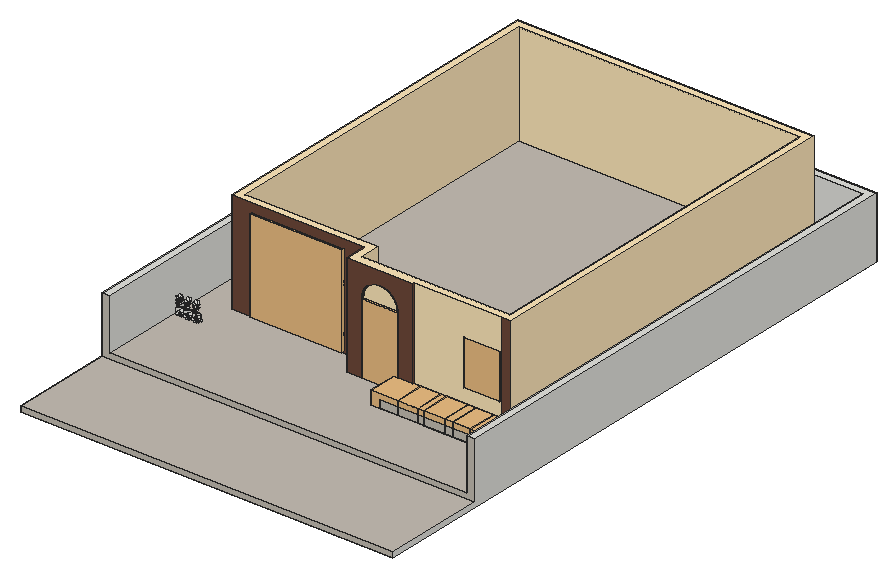
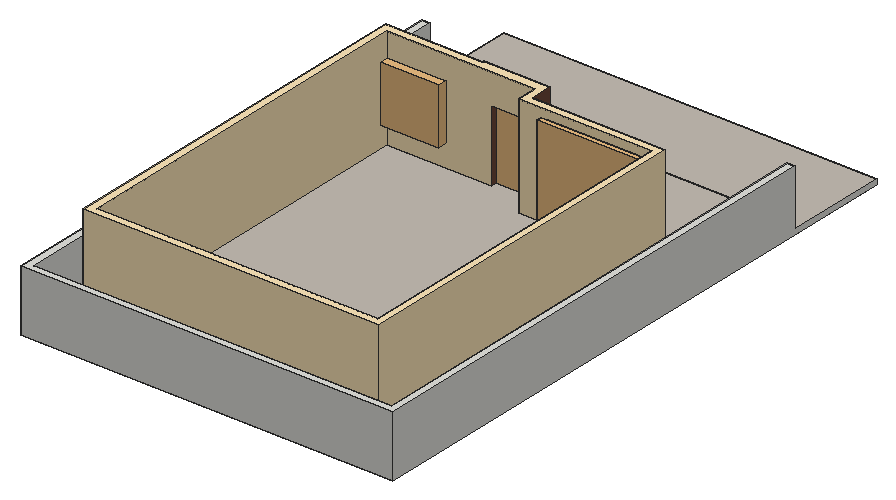
# SketchUp Ruby script. Lengths in inches.
U = 1.inch
M = Sketchup.active_model
def pt(a) = Geom::Point3d.new(a.map { |v| v * U })
def face(e, loops, mat)
  f = e.add_face(loops[0].map { |a| pt(a) })
  loops[1..].each { |l| e.add_face(l.map { |a| pt(a) }).erase! }
  f.material = f.back_material = mat if mat
  f
end
# faces: each face lists its corners as indices into pts; further lists are holes
def faces(e, pts, list, mat = nil) = list.each { |f| face(e, (f[0].is_a?(Array) ? f : [f]).map { |l| l.map { |i| pts[i] } }, mat) }
# xy, xz, yz: faces in a plane at the given z, y or x. An outline is a flat list of corners, or four numbers for a rectangle; further outlines are holes
def ring(l) = l.size == 4 ? [[l[0], l[1]], [l[2], l[1]], [l[2], l[3]], [l[0], l[3]]] : l.each_slice(2).to_a
def flat(e, list, mat, &to3) = list.each { |f| face(e, (f[0].is_a?(Array) ? f : [f]).map { |l| ring(l).map { |u, v| to3.(u, v) } }, mat) }
def xy(e, z, list, mat = nil) = flat(e, list, mat) { |x, y| [x, y, z] }
def xz(e, y, list, mat = nil) = flat(e, list, mat) { |x, z| [x, y, z] }
def yz(e, x, list, mat = nil) = flat(e, list, mat) { |y, z| [x, y, z] }
def lines(e, pts, list) = list.each { |a, b| e.add_line(pt(pts[a]), pt(pts[b])) }
# prism: a flat outline (further loops are holes) pulled along v
def prism(e, loops, v, mat = nil)
  f = face(e, loops, mat); d = Geom::Vector3d.new(v.map { |x| x * U })
  f.pushpull(f.normal.samedirection?(d) ? d.length : -d.length)
end
def box(e, o, s, mat = nil) = prism(e, [[o, [o[0] + s[0], o[1], o[2]], [o[0] + s[0], o[1] + s[1], o[2]], [o[0], o[1] + s[1], o[2]]]], [0, 0, s[2]], mat)
def at(x, y, z, deg = 0) = Geom::Transformation.translation(pt([x, y, z])) * Geom::Transformation.rotation(ORIGIN, Z_AXIS, deg.degrees)
def axes(o, x, y, z) = Geom::Transformation.new([*x, 0, *y, 0, *z, 0, *pt(o).to_a, 1])
def part(name) = M.definitions.add(name)
# library, detail: a bought-in or finely detailed component or shape, given as its bounding box
def library(name, o, s) = part(name).tap { |d| box(d.entities, o, s) }
def detail(e, o, s) = box(e.add_group.entities, o, s)
def put(e, d, t, mat = nil) = e.add_instance(d, t).tap { |i| i.material = mat if mat }
def group(e, t, mat = nil) = e.add_group.tap { |g| g.transformation = t; g.material = mat if mat }.entities
root = M.entities
M.materials.add("1026 AP 7946 SUNNY SIDE UP").color = [254, 231, 186]
M.materials.add("1916 AP K226 Macadamia Cream-N").color = [109, 72, 58]
M.materials.add("[Field Rectangle Tile]").color = [196, 189, 179]
M.materials.add("[Steel Brushed Stainless]").color = [48, 48, 48]
c1 = part("Component\#6")
p = [[0.01,0,0],[0,3.24,4.54],[4.32,3.24,4.54],[4.33,0,0]]
faces(c1.entities,p,[[0,1,2,3]])
c2 = library("porta 4",[0.2,-5.42,1.33],[46.55,4.72,83.21])
c3 = library("Glazed double door",[0,0,0],[5.31,78.43,99.16])
c4 = library("Curtains",[0,0,0],[101.19,6.19,107.53])
c5 = library("---------1\#1",[5.49,6.625,-77.21],[69.81,13.39,114.05])
c6 = library("Monstera",[-45.82,-31.79,6.14],[177.56,112.18,50.31])
c7 = library("Group\#26",[0,-3.33,0],[108,3.74,108])
xy(root,-12,[[0,0,438,710]])
xy(root,-6,[[0,0,438,120]],"[Field Rectangle Tile]")
xy(root,0,[[9,120,429,701]],"[Field Rectangle Tile]")
xy(root,60,[[0,120,9,120,9,701,429,701,429,120,438,120,438,710,0,710]])
xz(root,0,[[0,-12,438,-6]],"[Field Rectangle Tile]")
xz(root,120,[[0,-6,438,-6,438,60,429,60,429,0,9,0,9,60,0,60]],"[Field Rectangle Tile]")
xz(root,701,[[9,0,429,60]])
xz(root,710,[[0,-12,438,60]])
yz(root,0,[[0,-12,0,-6,120,-6,120,60,710,60,710,-12]])
yz(root,9,[[120,0,701,60]])
yz(root,429,[[120,0,701,60]])
yz(root,438,[[0,-12,710,-12,710,60,120,60,120,-6,0,-6]])
put(root,c1,axes([14.53,209.94,4.23],[-0.07499,0.16237,1.17608],[0.09639,1.17545,-0.15681],[1.25477,-0.08059,0.08234]))
put(root,c1,axes([28.31,209.94,4.23],[0.07499,0.16237,1.17608],[-0.09639,1.17545,-0.15681],[-1.25477,-0.08059,0.08234]))
put(root,c1,axes([24.34,209.94,4.23],[-0.07499,0.16237,1.17608],[0.09639,1.17545,-0.15681],[1.25477,-0.08059,0.08234]))
put(root,c1,axes([38.11,209.94,4.23],[0.07499,0.16237,1.17608],[-0.09639,1.17545,-0.15681],[-1.25477,-0.08059,0.08234]))
put(root,c1,axes([34.14,209.94,4.23],[-0.07499,0.16237,1.17608],[0.09639,1.17545,-0.15681],[1.25477,-0.08059,0.08234]))
put(root,c1,axes([14.53,211.25,18.13],[0.01725,0.58763,-0.23192],[-0.06908,-0.2292,-0.5853],[0.66607,-0.03899,-0.0547]))
put(root,c1,axes([18.5,211.25,18.13],[-0.01725,0.58763,-0.23192],[0.06908,-0.2292,-0.5853],[-0.66607,-0.03899,-0.0547]))
put(root,c1,axes([24.34,211.25,18.13],[0.01725,0.58763,-0.23192],[-0.06908,-0.2292,-0.5853],[0.66607,-0.03899,-0.0547]))
put(root,c1,axes([28.31,211.25,18.13],[-0.01725,0.58763,-0.23192],[0.06908,-0.2292,-0.5853],[-0.66607,-0.03899,-0.0547]))
put(root,c1,axes([34.14,211.25,18.13],[0.01725,0.58763,-0.23192],[-0.06908,-0.2292,-0.5853],[0.66607,-0.03899,-0.0547]))
put(root,c1,axes([38.11,211.25,18.13],[-0.01725,0.58763,-0.23192],[0.06908,-0.2292,-0.5853],[-0.66607,-0.03899,-0.0547]))
put(root,c1,axes([18.5,210.82,6.78],[-0.05791,0.63342,0.22945],[-0.07755,0.22326,-0.63376],[-0.7099,-0.07606,0.05052]))
put(root,c1,axes([28.31,210.82,6.78],[-0.05791,0.63342,0.22945],[-0.07755,0.22326,-0.63376],[-0.7099,-0.07606,0.05052]))
put(root,c1,axes([38.11,210.82,6.78],[-0.05791,0.63342,0.22945],[-0.07755,0.22326,-0.63376],[-0.7099,-0.07606,0.05052]))
put(root,c1,axes([14.53,210.82,6.78],[0.05791,0.63342,0.22945],[0.07755,0.22326,-0.63376],[0.7099,-0.07606,0.05052]))
put(root,c1,axes([24.34,210.82,6.78],[0.05791,0.63342,0.22945],[0.07755,0.22326,-0.63376],[0.7099,-0.07606,0.05052]))
put(root,c1,axes([34.14,210.82,6.78],[0.05791,0.63342,0.22945],[0.07755,0.22326,-0.63376],[0.7099,-0.07606,0.05052]))
put(root,c1,axes([18.5,213.68,13.61],[-0.09122,-0.87293,0.35057],[0.03759,0.34878,0.87716],[-0.99643,0.09307,0.001]))
put(root,c1,axes([18.5,213.68,16.94],[-0.09122,-0.87293,0.35057],[0.03759,0.34878,0.87716],[-0.99643,0.09307,0.001]))
put(root,c1,axes([14.53,213.68,13.61],[0.09122,-0.87293,0.35057],[-0.03759,0.34878,0.87716],[0.99643,0.09307,0.001]))
put(root,c1,axes([14.53,213.68,16.94],[0.09122,-0.87293,0.35057],[-0.03759,0.34878,0.87716],[0.99643,0.09307,0.001]))
put(root,c1,axes([28.31,213.68,13.61],[-0.09122,-0.87293,0.35057],[0.03759,0.34878,0.87716],[-0.99643,0.09307,0.001]))
put(root,c1,axes([28.31,213.68,16.94],[-0.09122,-0.87293,0.35057],[0.03759,0.34878,0.87716],[-0.99643,0.09307,0.001]))
put(root,c1,axes([24.34,213.68,13.61],[0.09122,-0.87293,0.35057],[-0.03759,0.34878,0.87716],[0.99643,0.09307,0.001]))
put(root,c1,axes([24.34,213.68,16.94],[0.09122,-0.87293,0.35057],[-0.03759,0.34878,0.87716],[0.99643,0.09307,0.001]))
put(root,c1,axes([38.11,213.68,13.61],[-0.09122,-0.87293,0.35057],[0.03759,0.34878,0.87716],[-0.99643,0.09307,0.001]))
put(root,c1,axes([38.11,213.68,16.94],[-0.09122,-0.87293,0.35057],[0.03759,0.34878,0.87716],[-0.99643,0.09307,0.001]))
put(root,c1,axes([34.14,213.68,13.61],[0.09122,-0.87293,0.35057],[-0.03759,0.34878,0.87716],[0.99643,0.09307,0.001]))
put(root,c1,axes([34.14,213.68,16.94],[0.09122,-0.87293,0.35057],[-0.03759,0.34878,0.87716],[0.99643,0.09307,0.001]))
put(root,c1,axes([18.5,210.81,4.97],[-0.03332,-0.20638,1.23099],[0.11506,1.22627,0.20836],[-1.31805,0.11226,-0.01293]))
put(root,c1,axes([14.53,210.81,4.97],[0.03332,-0.20638,1.23099],[-0.11506,1.22627,0.20836],[1.31805,0.11226,-0.01293]))
put(root,c1,axes([28.31,210.81,4.97],[-0.03332,-0.20638,1.23099],[0.11506,1.22627,0.20836],[-1.31805,0.11226,-0.01293]))
put(root,c1,axes([24.34,210.81,4.97],[0.03332,-0.20638,1.23099],[-0.11506,1.22627,0.20836],[1.31805,0.11226,-0.01293]))
put(root,c1,axes([38.11,210.81,4.97],[-0.03332,-0.20638,1.23099],[0.11506,1.22627,0.20836],[-1.31805,0.11226,-0.01293]))
put(root,c1,axes([34.14,210.81,4.97],[0.03332,-0.20638,1.23099],[-0.11506,1.22627,0.20836],[1.31805,0.11226,-0.01293]))
put(root,c1,axes([14.53,213.28,4.19],[0.08194,0.11028,-0.62172],[0.07302,-0.6241,-0.10214],[0.66532,0.05491,0.08778]))
put(root,c1,axes([18.5,213.28,4.19],[-0.08194,0.11028,-0.62172],[-0.07302,-0.6241,-0.10214],[-0.66532,0.05491,0.08778]))
put(root,c1,axes([24.34,213.28,4.19],[0.08194,0.11028,-0.62172],[0.07302,-0.6241,-0.10214],[0.66532,0.05491,0.08778]))
put(root,c1,axes([28.31,213.28,4.19],[-0.08194,0.11028,-0.62172],[-0.07302,-0.6241,-0.10214],[-0.66532,0.05491,0.08778]))
put(root,c1,axes([34.14,213.28,4.19],[0.08194,0.11028,-0.62172],[0.07302,-0.6241,-0.10214],[0.66532,0.05491,0.08778]))
put(root,c1,axes([38.11,213.28,4.19],[-0.08194,0.11028,-0.62172],[-0.07302,-0.6241,-0.10214],[-0.66532,0.05491,0.08778]))
put(root,c1,axes([14.53,211.49,4.24],[-0.12406,-0.24562,0.96087],[-0.14629,0.96216,0.22914],[1.04104,0.10594,0.1467]))
put(root,c1,axes([18.5,211.49,4.24],[0.12406,-0.24562,0.96087],[0.14629,0.96216,0.22914],[-1.04104,0.10594,0.1467]))
put(root,c1,axes([24.34,211.49,4.24],[-0.12406,-0.24562,0.96087],[-0.14629,0.96216,0.22914],[1.04104,0.10594,0.1467]))
put(root,c1,axes([28.31,211.49,4.24],[0.12406,-0.24562,0.96087],[0.14629,0.96216,0.22914],[-1.04104,0.10594,0.1467]))
put(root,c1,axes([34.14,211.49,4.24],[-0.12406,-0.24562,0.96087],[-0.14629,0.96216,0.22914],[1.04104,0.10594,0.1467]))
put(root,c1,axes([38.11,211.49,4.24],[0.12406,-0.24562,0.96087],[0.14629,0.96216,0.22914],[-1.04104,0.10594,0.1467]))
put(root,c1,axes([18.5,213.625,2.08],[-0.05814,-0.55559,0.66869],[-0.23916,0.65616,0.52668],[-0.88998,-0.14003,-0.18522]))
put(root,c1,axes([14.53,213.625,2.08],[0.05814,-0.55559,0.66869],[0.23916,0.65616,0.52668],[0.88998,-0.14003,-0.18522]))
put(root,c1,axes([28.31,213.625,2.08],[-0.05814,-0.55559,0.66869],[-0.23916,0.65616,0.52668],[-0.88998,-0.14003,-0.18522]))
put(root,c1,axes([24.34,213.625,2.08],[0.05814,-0.55559,0.66869],[0.23916,0.65616,0.52668],[0.88998,-0.14003,-0.18522]))
put(root,c1,axes([38.11,213.625,2.08],[-0.05814,-0.55559,0.66869],[-0.23916,0.65616,0.52668],[-0.88998,-0.14003,-0.18522]))
put(root,c1,axes([34.14,213.625,2.08],[0.05814,-0.55559,0.66869],[0.23916,0.65616,0.52668],[0.88998,-0.14003,-0.18522]))
put(root,c1,axes([19.18,214.43,20.82],[-0.40689,-0.33066,-0.61889],[-0.38957,-0.50621,0.4984],[-0.63361,0.52358,0.09101]))
put(root,c1,axes([13.86,214.43,20.82],[0.40689,-0.33066,-0.61889],[0.38957,-0.50621,0.4984],[0.63361,0.52358,0.09101]))
put(root,c1,axes([28.99,214.43,20.82],[-0.40689,-0.33066,-0.61889],[-0.38957,-0.50621,0.4984],[-0.63361,0.52358,0.09101]))
put(root,c1,axes([23.66,214.43,20.82],[0.40689,-0.33066,-0.61889],[0.38957,-0.50621,0.4984],[0.63361,0.52358,0.09101]))
put(root,c1,axes([38.79,214.43,20.82],[-0.40689,-0.33066,-0.61889],[-0.38957,-0.50621,0.4984],[-0.63361,0.52358,0.09101]))
put(root,c1,axes([33.47,214.43,20.82],[0.40689,-0.33066,-0.61889],[0.38957,-0.50621,0.4984],[0.63361,0.52358,0.09101]))
put(root,c1,axes([13.96,214.33,3.125],[0.1239,-0.08914,-0.58356],[0.39991,-0.44626,0.14373],[0.48128,0.39377,0.0308]))
put(root,c1,axes([19.08,214.33,3.125],[-0.1239,-0.08914,-0.58356],[-0.39991,-0.44626,0.14373],[-0.48128,0.39377,0.0308]))
put(root,c1,axes([23.77,214.33,3.125],[0.1239,-0.08914,-0.58356],[0.39991,-0.44626,0.14373],[0.48128,0.39377,0.0308]))
put(root,c1,axes([28.88,214.33,3.125],[-0.1239,-0.08914,-0.58356],[-0.39991,-0.44626,0.14373],[-0.48128,0.39377,0.0308]))
put(root,c1,axes([33.57,214.33,3.125],[0.1239,-0.08914,-0.58356],[0.39991,-0.44626,0.14373],[0.48128,0.39377,0.0308]))
put(root,c1,axes([38.69,214.33,3.125],[-0.1239,-0.08914,-0.58356],[-0.39991,-0.44626,0.14373],[-0.48128,0.39377,0.0308]))
put(root,c1,axes([18.66,213.9375,9.46],[0.03176,-0.01156,-1.03134],[-0.82675,-0.67538,-0.01509],[-0.71538,0.78001,-0.02835]))
put(root,c1,axes([14.375,213.9375,9.46],[-0.03176,-0.01156,-1.03134],[0.82675,-0.67538,-0.01509],[0.71538,0.78001,-0.02835]))
put(root,c1,axes([28.47,213.9375,9.46],[0.03176,-0.01156,-1.03134],[-0.82675,-0.67538,-0.01509],[-0.71538,0.78001,-0.02835]))
put(root,c1,axes([24.18,213.9375,9.46],[-0.03176,-0.01156,-1.03134],[0.82675,-0.67538,-0.01509],[0.71538,0.78001,-0.02835]))
put(root,c1,axes([38.27,213.9375,9.46],[0.03176,-0.01156,-1.03134],[-0.82675,-0.67538,-0.01509],[-0.71538,0.78001,-0.02835]))
put(root,c1,axes([33.99,213.9375,9.46],[-0.03176,-0.01156,-1.03134],[0.82675,-0.67538,-0.01509],[0.71538,0.78001,-0.02835]))
put(root,c1,axes([13.91,214.375,11.05],[-0.24885,0.08416,-0.78609],[0.48118,-0.65702,-0.20591],[0.6861,0.4913,-0.14071]))
put(root,c1,axes([19.125,214.375,11.05],[0.24885,0.08416,-0.78609],[-0.48118,-0.65702,-0.20591],[-0.6861,0.4913,-0.14071]))
put(root,c1,axes([23.72,214.375,11.05],[-0.24885,0.08416,-0.78609],[0.48118,-0.65702,-0.20591],[0.6861,0.4913,-0.14071]))
put(root,c1,axes([28.93,214.375,11.05],[0.24885,0.08416,-0.78609],[-0.48118,-0.65702,-0.20591],[-0.6861,0.4913,-0.14071]))
put(root,c1,axes([33.52,214.375,11.05],[-0.24885,0.08416,-0.78609],[0.48118,-0.65702,-0.20591],[0.6861,0.4913,-0.14071]))
put(root,c1,axes([38.74,214.375,11.05],[0.24885,0.08416,-0.78609],[-0.48118,-0.65702,-0.20591],[-0.6861,0.4913,-0.14071]))
put(root,c1,axes([19.32,214.56,5.98],[-0.23258,-0.01173,-1.12749],[-0.77314,-0.87447,0.15104],[-0.91146,0.74476,0.15959]))
put(root,c1,axes([13.72,214.56,5.98],[0.23258,-0.01173,-1.12749],[0.77314,-0.87447,0.15104],[0.91146,0.74476,0.15959]))
put(root,c1,axes([29.12,214.56,5.98],[-0.23258,-0.01173,-1.12749],[-0.77314,-0.87447,0.15104],[-0.91146,0.74476,0.15959]))
put(root,c1,axes([23.53,214.56,5.98],[0.23258,-0.01173,-1.12749],[0.77314,-0.87447,0.15104],[0.91146,0.74476,0.15959]))
put(root,c1,axes([38.93,214.56,5.98],[-0.23258,-0.01173,-1.12749],[-0.77314,-0.87447,0.15104],[-0.91146,0.74476,0.15959]))
put(root,c1,axes([33.33,214.56,5.98],[0.23258,-0.01173,-1.12749],[0.77314,-0.87447,0.15104],[0.91146,0.74476,0.15959]))
g1 = group(root,at(45,228,0),"1026 AP 7946 SUNNY SIDE UP")
xy(g1,0,[[156,0,156,26,0,26,0,446,348,446,348,2,234,2,234,0,216,0,216,11,339,11,339,437,9,437,9,35,165,35,165,11,174,11,174,0]])
xy(g1,2,[[24,26,132,35]])
xy(g1,30,[[292,2,334,11]])
xy(g1,84,[[174,2,216,11],[292,2,334,11]])
xy(g1,105,[[194.56,0,195,2],[195,0,195.44,2]],"1916 AP K226 Macadamia Cream-N")
xy(g1,110,[[24,26,132,35]])
xy(g1,120,[[[156,0,234,0,234,2,348,2,348,446,0,446,0,26,156,26],[165,11,165,35,9,35,9,437,339,437,339,11]]])
xz(g1,0,[[156,0,174,0,174,84.44,174.04,85.32,174.07,85.76,174.12,86.2,174.17,86.63,174.23,87.07,174.29,87.5,174.37,87.94,174.55,88.8,174.66,89.22,174.77,89.65,175.03,90.49,175.17,90.91,175.47,91.73,175.64,92.14,176,92.94,176.19,93.34,176.39,93.73,176.6,94.12,176.8125,94.5,177.04,94.88,177.27,95.25,177.51,95.62,178.01,96.34,178.27,96.7,178.54,97.04,178.82,97.39,179.1,97.72,179.39,98.05,179.69,98.375,180,98.69,180.31,99,180.625,99.31,180.95,99.61,181.28,99.9,181.61,100.18,181.96,100.46,182.3,100.73,182.66,100.99,183.38,101.49,183.75,101.73,184.12,101.96,184.5,102.1875,184.88,102.4,185.27,102.61,185.66,102.81,186.06,103,186.86,103.36,187.27,103.53,188.09,103.83,188.51,103.97,189.35,104.23,189.78,104.34,190.2,104.45,191.06,104.63,191.5,104.71,191.93,104.77,192.37,104.83,192.8,104.88,193.24,104.93,193.68,104.96,194.56,105,195.44,105,196.32,104.96,196.76,104.93,197.2,104.88,197.63,104.83,198.07,104.77,198.5,104.71,198.94,104.63,199.8,104.45,200.22,104.34,200.65,104.23,201.49,103.97,201.91,103.83,202.73,103.53,203.14,103.36,203.94,103,204.34,102.81,204.73,102.61,205.12,102.4,205.5,102.1875,205.88,101.96,206.25,101.73,206.62,101.49,207.34,100.99,207.7,100.73,208.04,100.46,208.39,100.18,208.72,99.9,209.05,99.61,209.375,99.31,209.69,99,210,98.69,210.31,98.375,210.61,98.05,210.9,97.72,211.18,97.39,211.46,97.04,211.73,96.7,211.99,96.34,212.49,95.62,212.73,95.25,212.96,94.88,213.1875,94.5,213.4,94.12,213.61,93.73,213.81,93.34,214,92.94,214.36,92.14,214.53,91.73,214.83,90.91,214.97,90.49,215.23,89.65,215.34,89.22,215.45,88.8,215.63,87.94,215.71,87.5,215.77,87.07,215.83,86.63,215.88,86.2,215.93,85.76,215.96,85.32,216,84.44,216,0,234,0,234,120,156,120]],"1916 AP K226 Macadamia Cream-N")
xz(g1,2,[[[234,0,336,120],[292,30,334,84]],[174,84,216,84,216,84.44,215.96,85.32,215.93,85.76,215.88,86.2,215.83,86.63,215.77,87.07,215.71,87.5,215.63,87.94,215.45,88.8,215.34,89.22,215.23,89.65,214.97,90.49,214.83,90.91,214.53,91.73,214.36,92.14,214,92.94,213.81,93.34,213.61,93.73,213.4,94.12,213.1875,94.5,212.96,94.88,212.73,95.25,212.49,95.62,211.99,96.34,211.73,96.7,211.46,97.04,211.18,97.39,210.9,97.72,210.61,98.05,210.31,98.375,210,98.69,209.69,99,209.375,99.31,209.05,99.61,208.72,99.9,208.39,100.18,208.04,100.46,207.7,100.73,207.34,100.99,206.62,101.49,206.25,101.73,205.88,101.96,205.5,102.1875,205.12,102.4,204.73,102.61,204.34,102.81,203.94,103,203.14,103.36,202.73,103.53,201.91,103.83,201.49,103.97,200.65,104.23,200.22,104.34,199.8,104.45,198.94,104.63,198.5,104.71,198.07,104.77,197.63,104.83,197.2,104.88,196.76,104.93,196.32,104.96,195.44,105,194.56,105,193.68,104.96,193.24,104.93,192.8,104.88,192.37,104.83,191.93,104.77,191.5,104.71,191.06,104.63,190.2,104.45,189.78,104.34,189.35,104.23,188.51,103.97,188.09,103.83,187.27,103.53,186.86,103.36,186.06,103,185.66,102.81,185.27,102.61,184.88,102.4,184.5,102.1875,184.12,101.96,183.75,101.73,183.38,101.49,182.66,100.99,182.3,100.73,181.96,100.46,181.61,100.18,181.28,99.9,180.95,99.61,180.625,99.31,180.31,99,180,98.69,179.69,98.375,179.39,98.05,179.1,97.72,178.82,97.39,178.54,97.04,178.27,96.7,178.01,96.34,177.51,95.62,177.27,95.25,177.04,94.88,176.8125,94.5,176.6,94.12,176.39,93.73,176.19,93.34,176,92.94,175.64,92.14,175.47,91.73,175.17,90.91,175.03,90.49,174.77,89.65,174.66,89.22,174.55,88.8,174.37,87.94,174.29,87.5,174.23,87.07,174.17,86.63,174.12,86.2,174.07,85.76,174.04,85.32,174,84.44]])
xz(g1,2,[[336,0,348,120]],"1916 AP K226 Macadamia Cream-N")
xz(g1,11,[[[165,0,165,120,339,120,339,0,216,0,216,84,174,84,174,0],[292,30,334,84]]])
xz(g1,26,[[[0,0,156,120],[24,2,132,110]]],"1916 AP K226 Macadamia Cream-N")
xz(g1,35,[[[9,0,165,120],[24,2,132,110]]])
xz(g1,437,[[9,0,339,120]])
xz(g1,446,[[0,0,348,120]])
yz(g1,0,[[26,0,446,120]])
yz(g1,9,[[35,0,437,120]])
yz(g1,24,[[26,2,35,110]])
yz(g1,132,[[26,2,35,110]])
yz(g1,156,[[0,0,26,120]],"1916 AP K226 Macadamia Cream-N")
yz(g1,165,[[11,0,35,120]])
yz(g1,174,[[0,0,11,84],[0,84,2,84.44]],"1916 AP K226 Macadamia Cream-N")
yz(g1,216,[[0,0,11,84],[0,84,2,84.44]],"1916 AP K226 Macadamia Cream-N")
yz(g1,234,[[0,0,2,120]],"1916 AP K226 Macadamia Cream-N")
yz(g1,292,[[2,30,11,84]])
yz(g1,334,[[2,30,11,84]])
yz(g1,339,[[11,0,437,120]])
yz(g1,348,[[2,0,446,120]])
p = [[174,2,84.44],[174.02,2,84.88],[174.02,0,84.88],[174,0,84.44],[215.98,2,84.88],[216,2,84.44],
  [216,0,84.44],[215.98,0,84.88],[174.04,2,85.32],[174.04,0,85.32],[215.96,2,85.32],[215.96,0,85.32],
  [174.07,2,85.76],[174.07,0,85.76],[215.93,2,85.76],[215.93,0,85.76],[174.12,2,86.2],[174.12,0,86.2],
  [215.88,2,86.2],[215.88,0,86.2],[174.17,2,86.63],[174.17,0,86.63],[215.83,2,86.63],[215.83,0,86.63],
  [174.23,2,87.07],[174.23,0,87.07],[215.77,2,87.07],[215.77,0,87.07],[174.29,2,87.5],[174.29,0,87.5],
  [215.71,2,87.5],[215.71,0,87.5],[174.37,2,87.94],[174.37,0,87.94],[215.63,2,87.94],[215.63,0,87.94],
  [174.46,2,88.37],[174.46,0,88.37],[215.54,2,88.37],[215.54,0,88.37],[174.55,2,88.8],[174.55,0,88.8],
  [215.45,2,88.8],[215.45,0,88.8],[174.66,2,89.22],[174.66,0,89.22],[215.34,2,89.22],[215.34,0,89.22],
  [174.77,2,89.65],[174.77,0,89.65],[215.23,2,89.65],[215.23,0,89.65],[174.9,2,90.07],[174.9,0,90.07],
  [215.1,2,90.07],[215.1,0,90.07],[175.03,2,90.49],[175.03,0,90.49],[214.97,2,90.49],[214.97,0,90.49],
  [175.17,2,90.91],[175.17,0,90.91],[214.83,2,90.91],[214.83,0,90.91],[175.32,2,91.32],[175.32,0,91.32],
  [214.68,2,91.32],[214.68,0,91.32],[175.47,2,91.73],[175.47,0,91.73],[214.53,2,91.73],[214.53,0,91.73],
  [175.64,2,92.14],[175.64,0,92.14],[214.36,2,92.14],[214.36,0,92.14],[175.82,2,92.54],[175.82,0,92.54],
  [214.18,2,92.54],[214.18,0,92.54],[176,2,92.94],[176,0,92.94],[214,2,92.94],[214,0,92.94],
  [176.19,2,93.34],[176.19,0,93.34],[213.81,2,93.34],[213.81,0,93.34],[176.39,2,93.73],[176.39,0,93.73],
  [213.61,2,93.73],[213.61,0,93.73],[176.6,2,94.12],[176.6,0,94.12],[213.4,2,94.12],[213.4,0,94.12],
  [176.8125,2,94.5],[176.8125,0,94.5],[213.1875,2,94.5],[213.1875,0,94.5],[177.04,2,94.88],[177.04,0,94.88],
  [212.96,2,94.88],[212.96,0,94.88],[177.27,2,95.25],[177.27,0,95.25],[212.73,2,95.25],[212.73,0,95.25],
  [177.51,2,95.62],[177.51,0,95.62],[212.49,2,95.62],[212.49,0,95.62],[177.76,2,95.98],[177.76,0,95.98],
  [212.24,2,95.98],[212.24,0,95.98],[178.01,2,96.34],[178.01,0,96.34],[211.99,2,96.34],[211.99,0,96.34],
  [178.27,2,96.7],[178.27,0,96.7],[211.73,2,96.7],[211.73,0,96.7],[178.54,2,97.04],[178.54,0,97.04],
  [211.46,2,97.04],[211.46,0,97.04],[178.82,2,97.39],[178.82,0,97.39],[211.18,2,97.39],[211.18,0,97.39],
  [179.1,2,97.72],[179.1,0,97.72],[210.9,2,97.72],[210.9,0,97.72],[179.39,2,98.05],[179.39,0,98.05],
  [210.61,2,98.05],[210.61,0,98.05],[179.69,2,98.375],[179.69,0,98.375],[210.31,2,98.375],[210.31,0,98.375],
  [180,2,98.69],[180,0,98.69],[210,2,98.69],[210,0,98.69],[180.31,2,99],[180.31,0,99],
  [209.69,2,99],[209.69,0,99],[180.625,2,99.31],[180.625,0,99.31],[209.375,2,99.31],[209.375,0,99.31],
  [180.95,2,99.61],[180.95,0,99.61],[209.05,2,99.61],[209.05,0,99.61],[181.28,2,99.9],[181.28,0,99.9],
  [208.72,2,99.9],[208.72,0,99.9],[181.61,2,100.18],[181.61,0,100.18],[208.39,2,100.18],[208.39,0,100.18],
  [181.96,2,100.46],[181.96,0,100.46],[208.04,2,100.46],[208.04,0,100.46],[182.3,2,100.73],[182.3,0,100.73],
  [207.7,2,100.73],[207.7,0,100.73],[182.66,2,100.99],[182.66,0,100.99],[207.34,2,100.99],[207.34,0,100.99],
  [183.02,2,101.24],[183.02,0,101.24],[206.98,2,101.24],[206.98,0,101.24],[183.38,2,101.49],[183.38,0,101.49],
  [206.62,2,101.49],[206.62,0,101.49],[183.75,2,101.73],[183.75,0,101.73],[206.25,2,101.73],[206.25,0,101.73],
  [184.12,2,101.96],[184.12,0,101.96],[205.88,2,101.96],[205.88,0,101.96],[184.5,2,102.1875],[184.5,0,102.1875],
  [205.5,2,102.1875],[205.5,0,102.1875],[184.88,2,102.4],[184.88,0,102.4],[205.12,2,102.4],[205.12,0,102.4],
  [185.27,2,102.61],[185.27,0,102.61],[204.73,2,102.61],[204.73,0,102.61],[185.66,2,102.81],[185.66,0,102.81],
  [204.34,2,102.81],[204.34,0,102.81],[186.06,2,103],[186.06,0,103],[203.94,2,103],[203.94,0,103],
  [186.46,2,103.18],[186.46,0,103.18],[203.54,2,103.18],[203.54,0,103.18],[186.86,2,103.36],[186.86,0,103.36],
  [203.14,2,103.36],[203.14,0,103.36],[187.27,2,103.53],[187.27,0,103.53],[202.73,2,103.53],[202.73,0,103.53],
  [187.68,2,103.68],[187.68,0,103.68],[202.32,2,103.68],[202.32,0,103.68],[188.09,2,103.83],[188.09,0,103.83],
  [201.91,2,103.83],[201.91,0,103.83],[188.51,2,103.97],[188.51,0,103.97],[201.49,2,103.97],[201.49,0,103.97],
  [188.93,2,104.1],[188.93,0,104.1],[201.07,2,104.1],[201.07,0,104.1],[189.35,2,104.23],[189.35,0,104.23],
  [200.65,2,104.23],[200.65,0,104.23],[189.78,2,104.34],[189.78,0,104.34],[200.22,2,104.34],[200.22,0,104.34],
  [190.2,2,104.45],[190.2,0,104.45],[199.8,2,104.45],[199.8,0,104.45],[190.63,2,104.54],[190.63,0,104.54],
  [199.37,2,104.54],[199.37,0,104.54],[191.06,2,104.63],[191.06,0,104.63],[198.94,2,104.63],[198.94,0,104.63],
  [191.5,2,104.71],[191.5,0,104.71],[198.5,2,104.71],[198.5,0,104.71],[191.93,2,104.77],[191.93,0,104.77],
  [198.07,2,104.77],[198.07,0,104.77],[192.37,2,104.83],[192.37,0,104.83],[192.8,2,104.88],[192.8,0,104.88],
  [197.2,2,104.88],[197.63,2,104.83],[197.63,0,104.83],[197.2,0,104.88],[193.24,2,104.93],[193.24,0,104.93],
  [193.68,2,104.96],[193.68,0,104.96],[196.32,2,104.96],[196.76,2,104.93],[196.76,0,104.93],[196.32,0,104.96],
  [194.12,2,104.98],[194.12,0,104.98],[194.56,2,105],[194.56,0,105],[195.44,2,105],[195.88,2,104.98],
  [195.88,0,104.98],[195.44,0,105]]
faces(g1,p,[[0,1,2,3],[4,5,6,7],[1,8,9,2],[10,4,7,11],[8,12,13,9],[14,10,11,15],[12,16,17,13],[18,14,15,19],
  [16,20,21,17],[22,18,19,23],[20,24,25,21],[26,22,23,27],[24,28,29,25],[30,26,27,31],[28,32,33,29],[34,30,31,35],
  [32,36,37,33],[38,34,35,39],[36,40,41,37],[42,38,39,43],[40,44,45,41],[46,42,43,47],[44,48,49,45],[50,46,47,51],
  [48,52,53,49],[54,50,51,55],[52,56,57,53],[58,54,55,59],[56,60,61,57],[62,58,59,63],[60,64,65,61],[66,62,63,67],
  [64,68,69,65],[70,66,67,71],[68,72,73,69],[74,70,71,75],[72,76,77,73],[78,74,75,79],[76,80,81,77],[82,78,79,83],
  [80,84,85,81],[86,82,83,87],[84,88,89,85],[90,86,87,91],[88,92,93,89],[94,90,91,95],[92,96,97,93],[98,94,95,99],
  [96,100,101,97],[102,98,99,103],[100,104,105,101],[106,102,103,107],[104,108,109,105],[110,106,107,111],[108,112,113,109],[114,110,111,115],
  [112,116,117,113],[118,114,115,119],[116,120,121,117],[122,118,119,123],[120,124,125,121],[126,122,123,127],[124,128,129,125],[130,126,127,131],
  [128,132,133,129],[134,130,131,135],[132,136,137,133],[138,134,135,139],[136,140,141,137],[142,138,139,143],[140,144,145,141],[146,142,143,147],
  [144,148,149,145],[150,146,147,151],[148,152,153,149],[154,150,151,155],[152,156,157,153],[158,154,155,159],[156,160,161,157],[162,158,159,163],
  [160,164,165,161],[166,162,163,167],[164,168,169,165],[170,166,167,171],[168,172,173,169],[174,170,171,175],[172,176,177,173],[178,174,175,179],
  [176,180,181,177],[182,178,179,183],[180,184,185,181],[186,182,183,187],[184,188,189,185],[190,186,187,191],[188,192,193,189],[194,190,191,195],
  [192,196,197,193],[198,194,195,199],[196,200,201,197],[202,198,199,203],[200,204,205,201],[206,202,203,207],[204,208,209,205],[210,206,207,211],
  [208,212,213,209],[214,210,211,215],[212,216,217,213],[218,214,215,219],[216,220,221,217],[222,218,219,223],[220,224,225,221],[226,222,223,227],
  [224,228,229,225],[230,226,227,231],[228,232,233,229],[234,230,231,235],[232,236,237,233],[238,234,235,239],[236,240,241,237],[242,238,239,243],
  [240,244,245,241],[246,242,243,247],[244,248,249,245],[250,246,247,251],[248,252,253,249],[254,250,251,255],[252,256,257,253],[258,254,255,259],
  [256,260,261,257],[262,258,259,263],[260,264,265,261],[266,262,263,267],[264,268,269,265],[270,266,267,271],[268,272,273,269],[272,274,275,273],
  [276,277,278,279],[277,270,271,278],[274,280,281,275],[280,282,283,281],[284,285,286,287],[285,276,279,286],[282,288,289,283],[288,290,291,289],
  [292,293,294,295],[293,284,287,294]],"1916 AP K226 Macadamia Cream-N")
put(g1,c2,axes([173.82,5.28,-1.36],[0.90228,0,0],[0,1,0],[0,0,1.00971]))
put(g1,c3,axes([292,8.31,30],[0,-1,0],[0.53554,0,0],[0,0,0.54459]))
put(g1,c4,axes([15,35,0],[1.221,0,0],[0,1,0],[0,0,1.02]))
put(g1,c5,axes([264.12,1.375,46.92],[1,0,0],[0,1,0],[0,0,-0.58]))
put(g1,c6,axes([225.83,-24.14,-1.9],[0.31,0,0],[0,0.31,0],[0,0,0.31]))
put(g1,c6,axes([257.33,-24.14,-1.9],[0.31,0,0],[0,0.31,0],[0,0,0.31]))
put(g1,c6,axes([287.77,-24.14,-1.9],[0.31,0,0],[0,0.31,0],[0,0,0.31]))
put(g1,c6,axes([321.83,-24.14,-1.9],[0.31,0,0],[0,0.31,0],[0,0,0.31]))
put(g1,c7,at(24,26,2),"[Steel Brushed Stainless]")
g2 = group(g1,at(234,2,0),"[Field Rectangle Tile]")
xy(g2,0,[[-12,-36,-12,-2,0,-2,0,0,102,0,102,-3,3,-3,3,-5,-9,-5,-9,-33,102,-33,102,-36],[102,-36,102,-33,111,-33,111,-3,102,-3,102,0,114,0,114,-36]])
xy(g2,3,[[-9,-33,111,-33,111,-3,3,-3,3,-5,-9,-5]])
xy(g2,9,[[[-12,-36,114,-36,114,0,0,0,0,-2,-12,-2],[-9,-33,-9,-5,3,-5,3,-3,111,-3,111,-33]]])
xz(g2,-36,[[-12,0,114,9]])
xz(g2,-33,[[-9,0,0,3],[0,0,102,3],[102,0,111,3],[-9,3,0,9],[0,3,102,9],
  [102,3,111,9]])
xz(g2,-5,[[-9,0,3,3],[-9,3,3,9]])
xz(g2,-3,[[3,0,102,3],[102,0,111,3],[3,3,102,9],[102,3,111,9]])
xz(g2,-2,[[-12,0,0,9]])
xz(g2,0,[[0,0,114,9]])
yz(g2,-12,[[-36,0,-2,9]])
yz(g2,-9,[[-33,0,-5,3],[-33,3,-5,9]])
yz(g2,0,[[-2,0,0,9]])
yz(g2,3,[[-5,0,-3,3],[-5,3,-3,9]])
yz(g2,111,[[-33,0,-3,3],[-33,3,-3,9]])
yz(g2,114,[[-36,0,0,9]])
